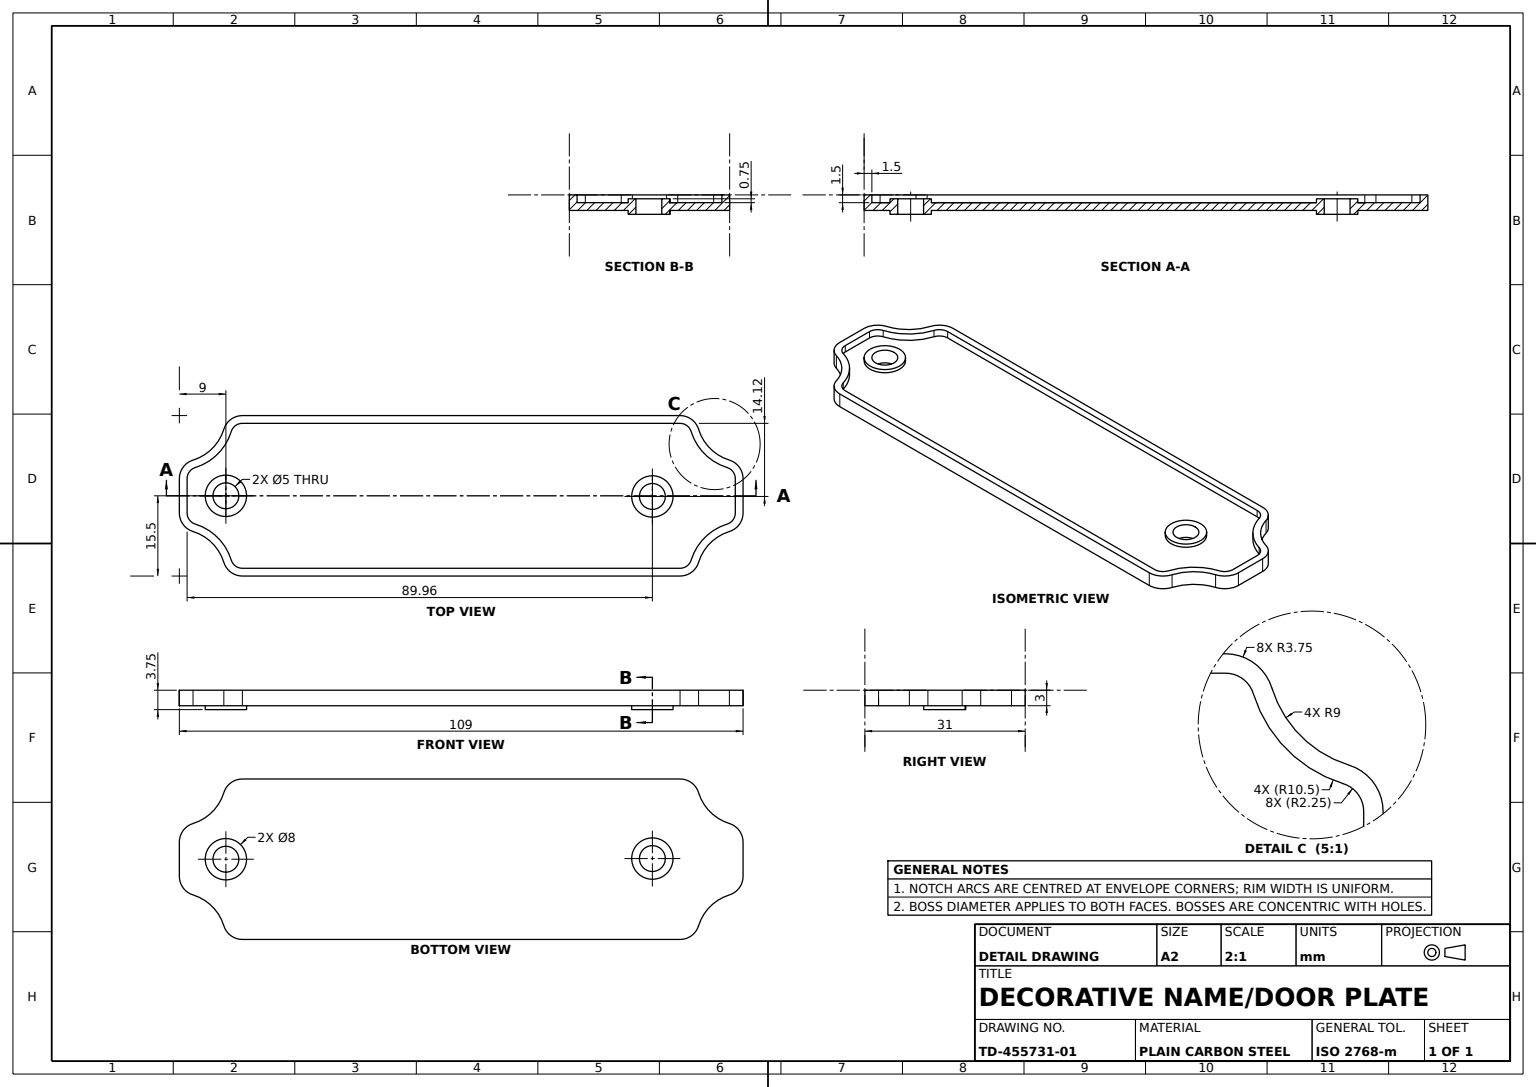
ISO-10303-21;
HEADER;
FILE_DESCRIPTION((''),'2;1');
FILE_NAME('','',(''),(''),'','','');
FILE_SCHEMA(('AUTOMOTIVE_DESIGN'));
ENDSEC;
DATA;
#1=APPLICATION_CONTEXT('');
#2=PRODUCT_CONTEXT('',#1,'mechanical');
#3=PRODUCT('','','',(#2));
#4=PRODUCT_DEFINITION_FORMATION('','',#3);
#5=PRODUCT_DEFINITION_CONTEXT('',#1,'design');
#6=PRODUCT_DEFINITION('','',#4,#5);
#7=PRODUCT_DEFINITION_SHAPE('','',#6);
#8=(LENGTH_UNIT()NAMED_UNIT(*)SI_UNIT(.MILLI.,.METRE.));
#9=(NAMED_UNIT(*)PLANE_ANGLE_UNIT()SI_UNIT($,.RADIAN.));
#10=(NAMED_UNIT(*)SI_UNIT($,.STERADIAN.)SOLID_ANGLE_UNIT());
#11=UNCERTAINTY_MEASURE_WITH_UNIT(LENGTH_MEASURE(1.E-05),#8,'distance_accuracy_value','');
#12=(GEOMETRIC_REPRESENTATION_CONTEXT(3)GLOBAL_UNCERTAINTY_ASSIGNED_CONTEXT((#11))GLOBAL_UNIT_ASSIGNED_CONTEXT((#8,#9,#10))REPRESENTATION_CONTEXT('',''));
#13=CARTESIAN_POINT('',(36.963445,-1.5,-3.876789));
#14=VERTEX_POINT('',#13);
#15=CARTESIAN_POINT('',(36.963445,-1.5,4.123211));
#16=VERTEX_POINT('',#15);
#17=CARTESIAN_POINT('',(36.963445,-1.5,0.123211));
#18=DIRECTION('',(0.,1.,0.));
#19=DIRECTION('',(0.,0.,1.));
#20=AXIS2_PLACEMENT_3D('',#17,#18,#19);
#21=CIRCLE('',#20,4.);
#22=EDGE_CURVE('',#14,#16,#21,.T.);
#23=ORIENTED_EDGE('',*,*,#22,.T.);
#24=EDGE_CURVE('',#16,#14,#21,.T.);
#25=ORIENTED_EDGE('',*,*,#24,.T.);
#26=EDGE_LOOP('',(#23,#25));
#27=FACE_BOUND('',#26,.T.);
#28=CARTESIAN_POINT('',(54.5,-1.5,-3.313942));
#29=VERTEX_POINT('',#28);
#30=CARTESIAN_POINT('',(51.852941,-1.5,-6.898077));
#31=VERTEX_POINT('',#30);
#32=CARTESIAN_POINT('',(50.75,-1.5,-3.313942));
#33=DIRECTION('',(0.,0.,-1.));
#34=AXIS2_PLACEMENT_3D('',#32,#18,#33);
#35=CIRCLE('',#34,3.75);
#36=EDGE_CURVE('',#29,#31,#35,.T.);
#37=ORIENTED_EDGE('',*,*,#36,.F.);
#38=CARTESIAN_POINT('',(54.5,-1.5,3.313942));
#39=VERTEX_POINT('',#38);
#40=VECTOR('',#33,1000.);
#41=LINE('',#28,#40);
#42=EDGE_CURVE('',#39,#29,#41,.T.);
#43=ORIENTED_EDGE('',*,*,#42,.F.);
#44=CARTESIAN_POINT('',(51.852941,-1.5,6.898077));
#45=VERTEX_POINT('',#44);
#46=CARTESIAN_POINT('',(50.75,-1.5,3.313942));
#47=AXIS2_PLACEMENT_3D('',#46,#18,#19);
#48=CIRCLE('',#47,3.75);
#49=EDGE_CURVE('',#45,#39,#48,.T.);
#50=ORIENTED_EDGE('',*,*,#49,.F.);
#51=CARTESIAN_POINT('',(45.898077,-1.5,12.852941));
#52=VERTEX_POINT('',#51);
#53=CARTESIAN_POINT('',(54.5,-1.5,15.5));
#54=DIRECTION('',(0.,-1.,0.));
#55=AXIS2_PLACEMENT_3D('',#53,#54,#19);
#56=CIRCLE('',#55,9.);
#57=EDGE_CURVE('',#52,#45,#56,.T.);
#58=ORIENTED_EDGE('',*,*,#57,.F.);
#59=CARTESIAN_POINT('',(42.313942,-1.5,15.5));
#60=VERTEX_POINT('',#59);
#61=CARTESIAN_POINT('',(42.313942,-1.5,11.75));
#62=AXIS2_PLACEMENT_3D('',#61,#18,#19);
#63=CIRCLE('',#62,3.75);
#64=EDGE_CURVE('',#60,#52,#63,.T.);
#65=ORIENTED_EDGE('',*,*,#64,.F.);
#66=CARTESIAN_POINT('',(-42.313942,-1.5,15.5));
#67=VERTEX_POINT('',#66);
#68=DIRECTION('',(1.,0.,0.));
#69=VECTOR('',#68,1000.);
#70=LINE('',#66,#69);
#71=EDGE_CURVE('',#67,#60,#70,.T.);
#72=ORIENTED_EDGE('',*,*,#71,.F.);
#73=CARTESIAN_POINT('',(-45.898077,-1.5,12.852941));
#74=VERTEX_POINT('',#73);
#75=CARTESIAN_POINT('',(-42.313942,-1.5,11.75));
#76=AXIS2_PLACEMENT_3D('',#75,#18,#19);
#77=CIRCLE('',#76,3.75);
#78=EDGE_CURVE('',#74,#67,#77,.T.);
#79=ORIENTED_EDGE('',*,*,#78,.F.);
#80=CARTESIAN_POINT('',(-51.852941,-1.5,6.898077));
#81=VERTEX_POINT('',#80);
#82=CARTESIAN_POINT('',(-54.5,-1.5,15.5));
#83=AXIS2_PLACEMENT_3D('',#82,#54,#19);
#84=CIRCLE('',#83,9.);
#85=EDGE_CURVE('',#81,#74,#84,.T.);
#86=ORIENTED_EDGE('',*,*,#85,.F.);
#87=CARTESIAN_POINT('',(-54.5,-1.5,3.313942));
#88=VERTEX_POINT('',#87);
#89=CARTESIAN_POINT('',(-50.75,-1.5,3.313942));
#90=AXIS2_PLACEMENT_3D('',#89,#18,#33);
#91=CIRCLE('',#90,3.75);
#92=EDGE_CURVE('',#88,#81,#91,.T.);
#93=ORIENTED_EDGE('',*,*,#92,.F.);
#94=CARTESIAN_POINT('',(-54.5,-1.5,-3.313942));
#95=VERTEX_POINT('',#94);
#96=VECTOR('',#19,1000.);
#97=LINE('',#94,#96);
#98=EDGE_CURVE('',#95,#88,#97,.T.);
#99=ORIENTED_EDGE('',*,*,#98,.F.);
#100=CARTESIAN_POINT('',(-51.852941,-1.5,-6.898077));
#101=VERTEX_POINT('',#100);
#102=CARTESIAN_POINT('',(-50.75,-1.5,-3.313942));
#103=AXIS2_PLACEMENT_3D('',#102,#18,#19);
#104=CIRCLE('',#103,3.75);
#105=EDGE_CURVE('',#101,#95,#104,.T.);
#106=ORIENTED_EDGE('',*,*,#105,.F.);
#107=CARTESIAN_POINT('',(-45.898077,-1.5,-12.852941));
#108=VERTEX_POINT('',#107);
#109=CARTESIAN_POINT('',(-54.5,-1.5,-15.5));
#110=AXIS2_PLACEMENT_3D('',#109,#54,#19);
#111=CIRCLE('',#110,9.);
#112=EDGE_CURVE('',#108,#101,#111,.T.);
#113=ORIENTED_EDGE('',*,*,#112,.F.);
#114=CARTESIAN_POINT('',(-42.313942,-1.5,-15.5));
#115=VERTEX_POINT('',#114);
#116=CARTESIAN_POINT('',(-42.313942,-1.5,-11.75));
#117=AXIS2_PLACEMENT_3D('',#116,#18,#19);
#118=CIRCLE('',#117,3.75);
#119=EDGE_CURVE('',#115,#108,#118,.T.);
#120=ORIENTED_EDGE('',*,*,#119,.F.);
#121=CARTESIAN_POINT('',(42.313942,-1.5,-15.5));
#122=VERTEX_POINT('',#121);
#123=DIRECTION('',(-1.,0.,0.));
#124=VECTOR('',#123,1000.);
#125=LINE('',#114,#124);
#126=EDGE_CURVE('',#122,#115,#125,.T.);
#127=ORIENTED_EDGE('',*,*,#126,.F.);
#128=CARTESIAN_POINT('',(45.898077,-1.5,-12.852941));
#129=VERTEX_POINT('',#128);
#130=CARTESIAN_POINT('',(42.313942,-1.5,-11.75));
#131=AXIS2_PLACEMENT_3D('',#130,#18,#19);
#132=CIRCLE('',#131,3.75);
#133=EDGE_CURVE('',#129,#122,#132,.T.);
#134=ORIENTED_EDGE('',*,*,#133,.F.);
#135=CARTESIAN_POINT('',(54.5,-1.5,-15.5));
#136=AXIS2_PLACEMENT_3D('',#135,#54,#19);
#137=CIRCLE('',#136,9.);
#138=EDGE_CURVE('',#31,#129,#137,.T.);
#139=ORIENTED_EDGE('',*,*,#138,.F.);
#140=EDGE_LOOP('',(#37,#43,#50,#58,#65,#72,#79,#86,#93,#99,#106,#113,#120,#127,#134,#139));
#141=FACE_OUTER_BOUND('',#140,.T.);
#142=CARTESIAN_POINT('',(-45.5,-1.5,-4.));
#143=VERTEX_POINT('',#142);
#144=CARTESIAN_POINT('',(-45.5,-1.5,4.));
#145=VERTEX_POINT('',#144);
#146=CARTESIAN_POINT('',(-45.5,-1.5,0.));
#147=AXIS2_PLACEMENT_3D('',#146,#18,#19);
#148=CIRCLE('',#147,4.);
#149=EDGE_CURVE('',#143,#145,#148,.T.);
#150=ORIENTED_EDGE('',*,*,#149,.T.);
#151=EDGE_CURVE('',#145,#143,#148,.T.);
#152=ORIENTED_EDGE('',*,*,#151,.T.);
#153=EDGE_LOOP('',(#150,#152));
#154=FACE_BOUND('',#153,.T.);
#155=PLANE('',#131);
#156=ADVANCED_FACE('',(#27,#141,#154),#155,.F.);
#157=CARTESIAN_POINT('',(-45.5,-2.25,2.5));
#158=VERTEX_POINT('',#157);
#159=CARTESIAN_POINT('',(-45.5,0.75,2.5));
#160=VERTEX_POINT('',#159);
#161=VECTOR('',#18,1000.);
#162=LINE('',#157,#161);
#163=EDGE_CURVE('',#158,#160,#162,.T.);
#164=ORIENTED_EDGE('',*,*,#163,.T.);
#165=CARTESIAN_POINT('',(-45.5,0.75,-2.5));
#166=VERTEX_POINT('',#165);
#167=CARTESIAN_POINT('',(-45.5,0.75,0.));
#168=AXIS2_PLACEMENT_3D('',#167,#18,#19);
#169=CIRCLE('',#168,2.5);
#170=EDGE_CURVE('',#160,#166,#169,.T.);
#171=ORIENTED_EDGE('',*,*,#170,.T.);
#172=CARTESIAN_POINT('',(-45.5,-2.25,-2.5));
#173=VERTEX_POINT('',#172);
#174=LINE('',#172,#161);
#175=EDGE_CURVE('',#173,#166,#174,.T.);
#176=ORIENTED_EDGE('',*,*,#175,.F.);
#177=CARTESIAN_POINT('',(-45.5,-2.25,0.));
#178=AXIS2_PLACEMENT_3D('',#177,#18,#19);
#179=CIRCLE('',#178,2.5);
#180=EDGE_CURVE('',#158,#173,#179,.T.);
#181=ORIENTED_EDGE('',*,*,#180,.F.);
#182=EDGE_LOOP('',(#164,#171,#176,#181));
#183=FACE_OUTER_BOUND('',#182,.T.);
#184=CYLINDRICAL_SURFACE('',#178,2.5);
#185=ADVANCED_FACE('',(#183),#184,.F.);
#186=CARTESIAN_POINT('',(-45.5,-2.25,-4.));
#187=VERTEX_POINT('',#186);
#188=CARTESIAN_POINT('',(-45.5,-2.25,4.));
#189=VERTEX_POINT('',#188);
#190=CIRCLE('',#178,4.);
#191=EDGE_CURVE('',#187,#189,#190,.T.);
#192=ORIENTED_EDGE('',*,*,#191,.F.);
#193=EDGE_CURVE('',#189,#187,#190,.T.);
#194=ORIENTED_EDGE('',*,*,#193,.F.);
#195=EDGE_LOOP('',(#192,#194));
#196=FACE_OUTER_BOUND('',#195,.T.);
#197=ORIENTED_EDGE('',*,*,#180,.T.);
#198=EDGE_CURVE('',#173,#158,#179,.T.);
#199=ORIENTED_EDGE('',*,*,#198,.T.);
#200=EDGE_LOOP('',(#197,#199));
#201=FACE_BOUND('',#200,.T.);
#202=PLANE('',#178);
#203=ADVANCED_FACE('',(#196,#201),#202,.F.);
#204=CARTESIAN_POINT('',(36.963445,-2.25,4.123211));
#205=VERTEX_POINT('',#204);
#206=CARTESIAN_POINT('',(36.963445,-2.25,-3.876789));
#207=VERTEX_POINT('',#206);
#208=CARTESIAN_POINT('',(36.963445,-2.25,0.123211));
#209=AXIS2_PLACEMENT_3D('',#208,#18,#19);
#210=CIRCLE('',#209,4.);
#211=EDGE_CURVE('',#205,#207,#210,.T.);
#212=ORIENTED_EDGE('',*,*,#211,.T.);
#213=LINE('',#206,#161);
#214=EDGE_CURVE('',#207,#14,#213,.T.);
#215=ORIENTED_EDGE('',*,*,#214,.T.);
#216=ORIENTED_EDGE('',*,*,#24,.F.);
#217=LINE('',#204,#161);
#218=EDGE_CURVE('',#205,#16,#217,.T.);
#219=ORIENTED_EDGE('',*,*,#218,.F.);
#220=EDGE_LOOP('',(#212,#215,#216,#219));
#221=FACE_OUTER_BOUND('',#220,.T.);
#222=CYLINDRICAL_SURFACE('',#209,4.);
#223=ADVANCED_FACE('',(#221),#222,.T.);
#224=CARTESIAN_POINT('',(-42.313942,1.5,-15.5));
#225=VERTEX_POINT('',#224);
#226=VECTOR('',#54,1000.);
#227=LINE('',#224,#226);
#228=EDGE_CURVE('',#225,#115,#227,.T.);
#229=ORIENTED_EDGE('',*,*,#228,.F.);
#230=CARTESIAN_POINT('',(42.313942,1.5,-15.5));
#231=VERTEX_POINT('',#230);
#232=LINE('',#224,#124);
#233=EDGE_CURVE('',#231,#225,#232,.T.);
#234=ORIENTED_EDGE('',*,*,#233,.F.);
#235=LINE('',#230,#226);
#236=EDGE_CURVE('',#231,#122,#235,.T.);
#237=ORIENTED_EDGE('',*,*,#236,.T.);
#238=ORIENTED_EDGE('',*,*,#126,.T.);
#239=EDGE_LOOP('',(#229,#234,#237,#238));
#240=FACE_OUTER_BOUND('',#239,.T.);
#241=AXIS2_PLACEMENT_3D('',#224,#19,#68);
#242=PLANE('',#241);
#243=ADVANCED_FACE('',(#240),#242,.F.);
#244=ORIENTED_EDGE('',*,*,#228,.T.);
#245=ORIENTED_EDGE('',*,*,#119,.T.);
#246=CARTESIAN_POINT('',(-45.898077,1.5,-12.852941));
#247=VERTEX_POINT('',#246);
#248=LINE('',#246,#226);
#249=EDGE_CURVE('',#247,#108,#248,.T.);
#250=ORIENTED_EDGE('',*,*,#249,.F.);
#251=CARTESIAN_POINT('',(-42.313942,1.5,-11.75));
#252=AXIS2_PLACEMENT_3D('',#251,#18,#19);
#253=CIRCLE('',#252,3.75);
#254=EDGE_CURVE('',#225,#247,#253,.T.);
#255=ORIENTED_EDGE('',*,*,#254,.F.);
#256=EDGE_LOOP('',(#244,#245,#250,#255));
#257=FACE_OUTER_BOUND('',#256,.T.);
#258=AXIS2_PLACEMENT_3D('',#251,#54,#33);
#259=CYLINDRICAL_SURFACE('',#258,3.75);
#260=ADVANCED_FACE('',(#257),#259,.T.);
#261=CARTESIAN_POINT('',(-53.,0.,-3.313942));
#262=VERTEX_POINT('',#261);
#263=CARTESIAN_POINT('',(-53.,1.5,-3.313942));
#264=VERTEX_POINT('',#263);
#265=LINE('',#261,#161);
#266=EDGE_CURVE('',#262,#264,#265,.T.);
#267=ORIENTED_EDGE('',*,*,#266,.T.);
#268=CARTESIAN_POINT('',(-53.,1.5,3.313942));
#269=VERTEX_POINT('',#268);
#270=LINE('',#263,#96);
#271=EDGE_CURVE('',#264,#269,#270,.T.);
#272=ORIENTED_EDGE('',*,*,#271,.T.);
#273=CARTESIAN_POINT('',(-53.,0.,3.313942));
#274=VERTEX_POINT('',#273);
#275=LINE('',#273,#161);
#276=EDGE_CURVE('',#274,#269,#275,.T.);
#277=ORIENTED_EDGE('',*,*,#276,.F.);
#278=LINE('',#261,#96);
#279=EDGE_CURVE('',#262,#274,#278,.T.);
#280=ORIENTED_EDGE('',*,*,#279,.F.);
#281=EDGE_LOOP('',(#267,#272,#277,#280));
#282=FACE_OUTER_BOUND('',#281,.T.);
#283=AXIS2_PLACEMENT_3D('',#261,#123,#19);
#284=PLANE('',#283);
#285=ADVANCED_FACE('',(#282),#284,.F.);
#286=CARTESIAN_POINT('',(36.963445,0.,-3.876789));
#287=VERTEX_POINT('',#286);
#288=CARTESIAN_POINT('',(36.963445,0.75,-3.876789));
#289=VERTEX_POINT('',#288);
#290=EDGE_CURVE('',#287,#289,#213,.T.);
#291=ORIENTED_EDGE('',*,*,#290,.T.);
#292=CARTESIAN_POINT('',(36.963445,0.75,4.123211));
#293=VERTEX_POINT('',#292);
#294=CARTESIAN_POINT('',(36.963445,0.75,0.123211));
#295=AXIS2_PLACEMENT_3D('',#294,#18,#19);
#296=CIRCLE('',#295,4.);
#297=EDGE_CURVE('',#293,#289,#296,.T.);
#298=ORIENTED_EDGE('',*,*,#297,.F.);
#299=CARTESIAN_POINT('',(36.963445,0.,4.123211));
#300=VERTEX_POINT('',#299);
#301=EDGE_CURVE('',#300,#293,#217,.T.);
#302=ORIENTED_EDGE('',*,*,#301,.F.);
#303=CARTESIAN_POINT('',(36.963445,0.,0.123211));
#304=AXIS2_PLACEMENT_3D('',#303,#18,#19);
#305=CIRCLE('',#304,4.);
#306=EDGE_CURVE('',#300,#287,#305,.T.);
#307=ORIENTED_EDGE('',*,*,#306,.T.);
#308=EDGE_LOOP('',(#291,#298,#302,#307));
#309=FACE_OUTER_BOUND('',#308,.T.);
#310=ADVANCED_FACE('',(#309),#222,.T.);
#311=EDGE_CURVE('',#289,#293,#296,.T.);
#312=ORIENTED_EDGE('',*,*,#311,.T.);
#313=ORIENTED_EDGE('',*,*,#297,.T.);
#314=EDGE_LOOP('',(#312,#313));
#315=FACE_OUTER_BOUND('',#314,.T.);
#316=CARTESIAN_POINT('',(36.963445,0.75,-2.376789));
#317=VERTEX_POINT('',#316);
#318=CARTESIAN_POINT('',(36.963445,0.75,2.623211));
#319=VERTEX_POINT('',#318);
#320=CIRCLE('',#295,2.5);
#321=EDGE_CURVE('',#317,#319,#320,.T.);
#322=ORIENTED_EDGE('',*,*,#321,.F.);
#323=EDGE_CURVE('',#319,#317,#320,.T.);
#324=ORIENTED_EDGE('',*,*,#323,.F.);
#325=EDGE_LOOP('',(#322,#324));
#326=FACE_BOUND('',#325,.T.);
#327=PLANE('',#295);
#328=ADVANCED_FACE('',(#315,#326),#327,.T.);
#329=ORIENTED_EDGE('',*,*,#311,.F.);
#330=ORIENTED_EDGE('',*,*,#290,.F.);
#331=EDGE_CURVE('',#287,#300,#305,.T.);
#332=ORIENTED_EDGE('',*,*,#331,.T.);
#333=ORIENTED_EDGE('',*,*,#301,.T.);
#334=EDGE_LOOP('',(#329,#330,#332,#333));
#335=FACE_OUTER_BOUND('',#334,.T.);
#336=ADVANCED_FACE('',(#335),#222,.T.);
#337=CARTESIAN_POINT('',(-42.313942,1.5,15.5));
#338=VERTEX_POINT('',#337);
#339=LINE('',#337,#226);
#340=EDGE_CURVE('',#338,#67,#339,.T.);
#341=ORIENTED_EDGE('',*,*,#340,.T.);
#342=ORIENTED_EDGE('',*,*,#71,.T.);
#343=CARTESIAN_POINT('',(42.313942,1.5,15.5));
#344=VERTEX_POINT('',#343);
#345=LINE('',#343,#226);
#346=EDGE_CURVE('',#344,#60,#345,.T.);
#347=ORIENTED_EDGE('',*,*,#346,.F.);
#348=LINE('',#337,#69);
#349=EDGE_CURVE('',#338,#344,#348,.T.);
#350=ORIENTED_EDGE('',*,*,#349,.F.);
#351=EDGE_LOOP('',(#341,#342,#347,#350));
#352=FACE_OUTER_BOUND('',#351,.T.);
#353=AXIS2_PLACEMENT_3D('',#337,#33,#123);
#354=PLANE('',#353);
#355=ADVANCED_FACE('',(#352),#354,.F.);
#356=CARTESIAN_POINT('',(53.,0.,-3.313942));
#357=VERTEX_POINT('',#356);
#358=CARTESIAN_POINT('',(53.,1.5,-3.313942));
#359=VERTEX_POINT('',#358);
#360=LINE('',#356,#161);
#361=EDGE_CURVE('',#357,#359,#360,.T.);
#362=ORIENTED_EDGE('',*,*,#361,.F.);
#363=CARTESIAN_POINT('',(53.,0.,3.313942));
#364=VERTEX_POINT('',#363);
#365=LINE('',#363,#40);
#366=EDGE_CURVE('',#364,#357,#365,.T.);
#367=ORIENTED_EDGE('',*,*,#366,.F.);
#368=CARTESIAN_POINT('',(53.,1.5,3.313942));
#369=VERTEX_POINT('',#368);
#370=LINE('',#363,#161);
#371=EDGE_CURVE('',#364,#369,#370,.T.);
#372=ORIENTED_EDGE('',*,*,#371,.T.);
#373=LINE('',#368,#40);
#374=EDGE_CURVE('',#369,#359,#373,.T.);
#375=ORIENTED_EDGE('',*,*,#374,.T.);
#376=EDGE_LOOP('',(#362,#367,#372,#375));
#377=FACE_OUTER_BOUND('',#376,.T.);
#378=AXIS2_PLACEMENT_3D('',#363,#68,#33);
#379=PLANE('',#378);
#380=ADVANCED_FACE('',(#377),#379,.F.);
#381=CARTESIAN_POINT('',(-51.852941,1.5,-6.898077));
#382=VERTEX_POINT('',#381);
#383=CARTESIAN_POINT('',(-54.5,1.5,-3.313942));
#384=VERTEX_POINT('',#383);
#385=CARTESIAN_POINT('',(-50.75,1.5,-3.313942));
#386=AXIS2_PLACEMENT_3D('',#385,#18,#19);
#387=CIRCLE('',#386,3.75);
#388=EDGE_CURVE('',#382,#384,#387,.T.);
#389=ORIENTED_EDGE('',*,*,#388,.T.);
#390=CARTESIAN_POINT('',(-54.5,1.5,3.313942));
#391=VERTEX_POINT('',#390);
#392=LINE('',#383,#96);
#393=EDGE_CURVE('',#384,#391,#392,.T.);
#394=ORIENTED_EDGE('',*,*,#393,.T.);
#395=CARTESIAN_POINT('',(-51.852941,1.5,6.898077));
#396=VERTEX_POINT('',#395);
#397=CARTESIAN_POINT('',(-50.75,1.5,3.313942));
#398=AXIS2_PLACEMENT_3D('',#397,#18,#33);
#399=CIRCLE('',#398,3.75);
#400=EDGE_CURVE('',#391,#396,#399,.T.);
#401=ORIENTED_EDGE('',*,*,#400,.T.);
#402=CARTESIAN_POINT('',(-45.898077,1.5,12.852941));
#403=VERTEX_POINT('',#402);
#404=CARTESIAN_POINT('',(-54.5,1.5,15.5));
#405=AXIS2_PLACEMENT_3D('',#404,#54,#19);
#406=CIRCLE('',#405,9.);
#407=EDGE_CURVE('',#396,#403,#406,.T.);
#408=ORIENTED_EDGE('',*,*,#407,.T.);
#409=CARTESIAN_POINT('',(-42.313942,1.5,11.75));
#410=AXIS2_PLACEMENT_3D('',#409,#18,#19);
#411=CIRCLE('',#410,3.75);
#412=EDGE_CURVE('',#403,#338,#411,.T.);
#413=ORIENTED_EDGE('',*,*,#412,.T.);
#414=ORIENTED_EDGE('',*,*,#349,.T.);
#415=CARTESIAN_POINT('',(45.898077,1.5,12.852941));
#416=VERTEX_POINT('',#415);
#417=CARTESIAN_POINT('',(42.313942,1.5,11.75));
#418=AXIS2_PLACEMENT_3D('',#417,#18,#19);
#419=CIRCLE('',#418,3.75);
#420=EDGE_CURVE('',#344,#416,#419,.T.);
#421=ORIENTED_EDGE('',*,*,#420,.T.);
#422=CARTESIAN_POINT('',(51.852941,1.5,6.898077));
#423=VERTEX_POINT('',#422);
#424=CARTESIAN_POINT('',(54.5,1.5,15.5));
#425=AXIS2_PLACEMENT_3D('',#424,#54,#19);
#426=CIRCLE('',#425,9.);
#427=EDGE_CURVE('',#416,#423,#426,.T.);
#428=ORIENTED_EDGE('',*,*,#427,.T.);
#429=CARTESIAN_POINT('',(54.5,1.5,3.313942));
#430=VERTEX_POINT('',#429);
#431=CARTESIAN_POINT('',(50.75,1.5,3.313942));
#432=AXIS2_PLACEMENT_3D('',#431,#18,#19);
#433=CIRCLE('',#432,3.75);
#434=EDGE_CURVE('',#423,#430,#433,.T.);
#435=ORIENTED_EDGE('',*,*,#434,.T.);
#436=CARTESIAN_POINT('',(54.5,1.5,-3.313942));
#437=VERTEX_POINT('',#436);
#438=LINE('',#436,#40);
#439=EDGE_CURVE('',#430,#437,#438,.T.);
#440=ORIENTED_EDGE('',*,*,#439,.T.);
#441=CARTESIAN_POINT('',(51.852941,1.5,-6.898077));
#442=VERTEX_POINT('',#441);
#443=CARTESIAN_POINT('',(50.75,1.5,-3.313942));
#444=AXIS2_PLACEMENT_3D('',#443,#18,#33);
#445=CIRCLE('',#444,3.75);
#446=EDGE_CURVE('',#437,#442,#445,.T.);
#447=ORIENTED_EDGE('',*,*,#446,.T.);
#448=CARTESIAN_POINT('',(45.898077,1.5,-12.852941));
#449=VERTEX_POINT('',#448);
#450=CARTESIAN_POINT('',(54.5,1.5,-15.5));
#451=AXIS2_PLACEMENT_3D('',#450,#54,#19);
#452=CIRCLE('',#451,9.);
#453=EDGE_CURVE('',#442,#449,#452,.T.);
#454=ORIENTED_EDGE('',*,*,#453,.T.);
#455=CARTESIAN_POINT('',(42.313942,1.5,-11.75));
#456=AXIS2_PLACEMENT_3D('',#455,#18,#19);
#457=CIRCLE('',#456,3.75);
#458=EDGE_CURVE('',#449,#231,#457,.T.);
#459=ORIENTED_EDGE('',*,*,#458,.T.);
#460=ORIENTED_EDGE('',*,*,#233,.T.);
#461=ORIENTED_EDGE('',*,*,#254,.T.);
#462=CARTESIAN_POINT('',(-54.5,1.5,-15.5));
#463=AXIS2_PLACEMENT_3D('',#462,#54,#19);
#464=CIRCLE('',#463,9.);
#465=EDGE_CURVE('',#247,#382,#464,.T.);
#466=ORIENTED_EDGE('',*,*,#465,.T.);
#467=EDGE_LOOP('',(#389,#394,#401,#408,#413,#414,#421,#428,#435,#440,#447,#454,#459,#460,#461,#466));
#468=FACE_OUTER_BOUND('',#467,.T.);
#469=CARTESIAN_POINT('',(-51.411765,1.5,5.464423));
#470=VERTEX_POINT('',#469);
#471=AXIS2_PLACEMENT_3D('',#397,#18,#19);
#472=CIRCLE('',#471,2.25);
#473=EDGE_CURVE('',#269,#470,#472,.T.);
#474=ORIENTED_EDGE('',*,*,#473,.F.);
#475=ORIENTED_EDGE('',*,*,#271,.F.);
#476=CARTESIAN_POINT('',(-51.411765,1.5,-5.464423));
#477=VERTEX_POINT('',#476);
#478=CIRCLE('',#386,2.25);
#479=EDGE_CURVE('',#477,#264,#478,.T.);
#480=ORIENTED_EDGE('',*,*,#479,.F.);
#481=CARTESIAN_POINT('',(-44.464423,1.5,-12.411765));
#482=VERTEX_POINT('',#481);
#483=CIRCLE('',#463,10.5);
#484=EDGE_CURVE('',#482,#477,#483,.T.);
#485=ORIENTED_EDGE('',*,*,#484,.F.);
#486=CARTESIAN_POINT('',(-42.313942,1.5,-14.));
#487=VERTEX_POINT('',#486);
#488=CIRCLE('',#252,2.25);
#489=EDGE_CURVE('',#487,#482,#488,.T.);
#490=ORIENTED_EDGE('',*,*,#489,.F.);
#491=CARTESIAN_POINT('',(42.313942,1.5,-14.));
#492=VERTEX_POINT('',#491);
#493=LINE('',#491,#124);
#494=EDGE_CURVE('',#492,#487,#493,.T.);
#495=ORIENTED_EDGE('',*,*,#494,.F.);
#496=CARTESIAN_POINT('',(44.464423,1.5,-12.411765));
#497=VERTEX_POINT('',#496);
#498=CIRCLE('',#456,2.25);
#499=EDGE_CURVE('',#497,#492,#498,.T.);
#500=ORIENTED_EDGE('',*,*,#499,.F.);
#501=CARTESIAN_POINT('',(51.411765,1.5,-5.464423));
#502=VERTEX_POINT('',#501);
#503=CIRCLE('',#451,10.5);
#504=EDGE_CURVE('',#502,#497,#503,.T.);
#505=ORIENTED_EDGE('',*,*,#504,.F.);
#506=AXIS2_PLACEMENT_3D('',#443,#18,#19);
#507=CIRCLE('',#506,2.25);
#508=EDGE_CURVE('',#359,#502,#507,.T.);
#509=ORIENTED_EDGE('',*,*,#508,.F.);
#510=ORIENTED_EDGE('',*,*,#374,.F.);
#511=CARTESIAN_POINT('',(51.411765,1.5,5.464423));
#512=VERTEX_POINT('',#511);
#513=CIRCLE('',#432,2.25);
#514=EDGE_CURVE('',#512,#369,#513,.T.);
#515=ORIENTED_EDGE('',*,*,#514,.F.);
#516=CARTESIAN_POINT('',(44.464423,1.5,12.411765));
#517=VERTEX_POINT('',#516);
#518=CIRCLE('',#425,10.5);
#519=EDGE_CURVE('',#517,#512,#518,.T.);
#520=ORIENTED_EDGE('',*,*,#519,.F.);
#521=CARTESIAN_POINT('',(42.313942,1.5,14.));
#522=VERTEX_POINT('',#521);
#523=CIRCLE('',#418,2.25);
#524=EDGE_CURVE('',#522,#517,#523,.T.);
#525=ORIENTED_EDGE('',*,*,#524,.F.);
#526=CARTESIAN_POINT('',(-42.313942,1.5,14.));
#527=VERTEX_POINT('',#526);
#528=LINE('',#526,#69);
#529=EDGE_CURVE('',#527,#522,#528,.T.);
#530=ORIENTED_EDGE('',*,*,#529,.F.);
#531=CARTESIAN_POINT('',(-44.464423,1.5,12.411765));
#532=VERTEX_POINT('',#531);
#533=CIRCLE('',#410,2.25);
#534=EDGE_CURVE('',#532,#527,#533,.T.);
#535=ORIENTED_EDGE('',*,*,#534,.F.);
#536=CIRCLE('',#405,10.5);
#537=EDGE_CURVE('',#470,#532,#536,.T.);
#538=ORIENTED_EDGE('',*,*,#537,.F.);
#539=EDGE_LOOP('',(#474,#475,#480,#485,#490,#495,#500,#505,#509,#510,#515,#520,#525,#530,#535,#538));
#540=FACE_BOUND('',#539,.T.);
#541=PLANE('',#456);
#542=ADVANCED_FACE('',(#468,#540),#541,.T.);
#543=ORIENTED_EDGE('',*,*,#439,.F.);
#544=LINE('',#429,#226);
#545=EDGE_CURVE('',#430,#39,#544,.T.);
#546=ORIENTED_EDGE('',*,*,#545,.T.);
#547=ORIENTED_EDGE('',*,*,#42,.T.);
#548=LINE('',#436,#226);
#549=EDGE_CURVE('',#437,#29,#548,.T.);
#550=ORIENTED_EDGE('',*,*,#549,.F.);
#551=EDGE_LOOP('',(#543,#546,#547,#550));
#552=FACE_OUTER_BOUND('',#551,.T.);
#553=AXIS2_PLACEMENT_3D('',#436,#123,#19);
#554=PLANE('',#553);
#555=ADVANCED_FACE('',(#552),#554,.F.);
#556=CARTESIAN_POINT('',(-44.464423,0.,-12.411765));
#557=VERTEX_POINT('',#556);
#558=LINE('',#556,#161);
#559=EDGE_CURVE('',#557,#482,#558,.T.);
#560=ORIENTED_EDGE('',*,*,#559,.T.);
#561=ORIENTED_EDGE('',*,*,#484,.T.);
#562=CARTESIAN_POINT('',(-51.411765,0.,-5.464423));
#563=VERTEX_POINT('',#562);
#564=LINE('',#562,#161);
#565=EDGE_CURVE('',#563,#477,#564,.T.);
#566=ORIENTED_EDGE('',*,*,#565,.F.);
#567=CARTESIAN_POINT('',(-54.5,0.,-15.5));
#568=AXIS2_PLACEMENT_3D('',#567,#54,#19);
#569=CIRCLE('',#568,10.5);
#570=EDGE_CURVE('',#557,#563,#569,.T.);
#571=ORIENTED_EDGE('',*,*,#570,.F.);
#572=EDGE_LOOP('',(#560,#561,#566,#571));
#573=FACE_OUTER_BOUND('',#572,.T.);
#574=AXIS2_PLACEMENT_3D('',#567,#18,#19);
#575=CYLINDRICAL_SURFACE('',#574,10.5);
#576=ADVANCED_FACE('',(#573),#575,.T.);
#577=ORIENTED_EDGE('',*,*,#524,.T.);
#578=CARTESIAN_POINT('',(44.464423,0.,12.411765));
#579=VERTEX_POINT('',#578);
#580=LINE('',#578,#161);
#581=EDGE_CURVE('',#579,#517,#580,.T.);
#582=ORIENTED_EDGE('',*,*,#581,.F.);
#583=CARTESIAN_POINT('',(42.313942,0.,14.));
#584=VERTEX_POINT('',#583);
#585=CARTESIAN_POINT('',(42.313942,0.,11.75));
#586=AXIS2_PLACEMENT_3D('',#585,#18,#19);
#587=CIRCLE('',#586,2.25);
#588=EDGE_CURVE('',#584,#579,#587,.T.);
#589=ORIENTED_EDGE('',*,*,#588,.F.);
#590=LINE('',#583,#161);
#591=EDGE_CURVE('',#584,#522,#590,.T.);
#592=ORIENTED_EDGE('',*,*,#591,.T.);
#593=EDGE_LOOP('',(#577,#582,#589,#592));
#594=FACE_OUTER_BOUND('',#593,.T.);
#595=CYLINDRICAL_SURFACE('',#586,2.25);
#596=ADVANCED_FACE('',(#594),#595,.F.);
#597=CARTESIAN_POINT('',(-45.5,0.,4.));
#598=VERTEX_POINT('',#597);
#599=CARTESIAN_POINT('',(-45.5,0.75,4.));
#600=VERTEX_POINT('',#599);
#601=LINE('',#188,#161);
#602=EDGE_CURVE('',#598,#600,#601,.T.);
#603=ORIENTED_EDGE('',*,*,#602,.F.);
#604=CARTESIAN_POINT('',(-45.5,0.,-4.));
#605=VERTEX_POINT('',#604);
#606=CARTESIAN_POINT('',(-45.5,0.,0.));
#607=AXIS2_PLACEMENT_3D('',#606,#18,#19);
#608=CIRCLE('',#607,4.);
#609=EDGE_CURVE('',#598,#605,#608,.T.);
#610=ORIENTED_EDGE('',*,*,#609,.T.);
#611=CARTESIAN_POINT('',(-45.5,0.75,-4.));
#612=VERTEX_POINT('',#611);
#613=LINE('',#186,#161);
#614=EDGE_CURVE('',#605,#612,#613,.T.);
#615=ORIENTED_EDGE('',*,*,#614,.T.);
#616=CIRCLE('',#168,4.);
#617=EDGE_CURVE('',#600,#612,#616,.T.);
#618=ORIENTED_EDGE('',*,*,#617,.F.);
#619=EDGE_LOOP('',(#603,#610,#615,#618));
#620=FACE_OUTER_BOUND('',#619,.T.);
#621=CYLINDRICAL_SURFACE('',#178,4.);
#622=ADVANCED_FACE('',(#620),#621,.T.);
#623=ORIENTED_EDGE('',*,*,#85,.T.);
#624=LINE('',#402,#226);
#625=EDGE_CURVE('',#403,#74,#624,.T.);
#626=ORIENTED_EDGE('',*,*,#625,.F.);
#627=ORIENTED_EDGE('',*,*,#407,.F.);
#628=LINE('',#395,#226);
#629=EDGE_CURVE('',#396,#81,#628,.T.);
#630=ORIENTED_EDGE('',*,*,#629,.T.);
#631=EDGE_LOOP('',(#623,#626,#627,#630));
#632=FACE_OUTER_BOUND('',#631,.T.);
#633=AXIS2_PLACEMENT_3D('',#404,#54,#33);
#634=CYLINDRICAL_SURFACE('',#633,9.);
#635=ADVANCED_FACE('',(#632),#634,.F.);
#636=LINE('',#448,#226);
#637=EDGE_CURVE('',#449,#129,#636,.T.);
#638=ORIENTED_EDGE('',*,*,#637,.T.);
#639=ORIENTED_EDGE('',*,*,#133,.T.);
#640=ORIENTED_EDGE('',*,*,#236,.F.);
#641=ORIENTED_EDGE('',*,*,#458,.F.);
#642=EDGE_LOOP('',(#638,#639,#640,#641));
#643=FACE_OUTER_BOUND('',#642,.T.);
#644=AXIS2_PLACEMENT_3D('',#455,#54,#33);
#645=CYLINDRICAL_SURFACE('',#644,3.75);
#646=ADVANCED_FACE('',(#643),#645,.T.);
#647=ORIENTED_EDGE('',*,*,#446,.F.);
#648=ORIENTED_EDGE('',*,*,#549,.T.);
#649=ORIENTED_EDGE('',*,*,#36,.T.);
#650=LINE('',#441,#226);
#651=EDGE_CURVE('',#442,#31,#650,.T.);
#652=ORIENTED_EDGE('',*,*,#651,.F.);
#653=EDGE_LOOP('',(#647,#648,#649,#652));
#654=FACE_OUTER_BOUND('',#653,.T.);
#655=AXIS2_PLACEMENT_3D('',#443,#54,#33);
#656=CYLINDRICAL_SURFACE('',#655,3.75);
#657=ADVANCED_FACE('',(#654),#656,.T.);
#658=EDGE_CURVE('',#187,#143,#613,.T.);
#659=ORIENTED_EDGE('',*,*,#658,.F.);
#660=ORIENTED_EDGE('',*,*,#191,.T.);
#661=EDGE_CURVE('',#189,#145,#601,.T.);
#662=ORIENTED_EDGE('',*,*,#661,.T.);
#663=ORIENTED_EDGE('',*,*,#149,.F.);
#664=EDGE_LOOP('',(#659,#660,#662,#663));
#665=FACE_OUTER_BOUND('',#664,.T.);
#666=ADVANCED_FACE('',(#665),#621,.T.);
#667=CARTESIAN_POINT('',(51.411765,0.,5.464423));
#668=VERTEX_POINT('',#667);
#669=CARTESIAN_POINT('',(54.5,0.,15.5));
#670=AXIS2_PLACEMENT_3D('',#669,#54,#19);
#671=CIRCLE('',#670,10.5);
#672=EDGE_CURVE('',#579,#668,#671,.T.);
#673=ORIENTED_EDGE('',*,*,#672,.F.);
#674=ORIENTED_EDGE('',*,*,#581,.T.);
#675=ORIENTED_EDGE('',*,*,#519,.T.);
#676=LINE('',#667,#161);
#677=EDGE_CURVE('',#668,#512,#676,.T.);
#678=ORIENTED_EDGE('',*,*,#677,.F.);
#679=EDGE_LOOP('',(#673,#674,#675,#678));
#680=FACE_OUTER_BOUND('',#679,.T.);
#681=AXIS2_PLACEMENT_3D('',#669,#18,#19);
#682=CYLINDRICAL_SURFACE('',#681,10.5);
#683=ADVANCED_FACE('',(#680),#682,.T.);
#684=CARTESIAN_POINT('',(51.411765,0.,-5.464423));
#685=VERTEX_POINT('',#684);
#686=CARTESIAN_POINT('',(50.75,0.,-3.313942));
#687=AXIS2_PLACEMENT_3D('',#686,#18,#19);
#688=CIRCLE('',#687,2.25);
#689=EDGE_CURVE('',#357,#685,#688,.T.);
#690=ORIENTED_EDGE('',*,*,#689,.F.);
#691=ORIENTED_EDGE('',*,*,#361,.T.);
#692=ORIENTED_EDGE('',*,*,#508,.T.);
#693=LINE('',#684,#161);
#694=EDGE_CURVE('',#685,#502,#693,.T.);
#695=ORIENTED_EDGE('',*,*,#694,.F.);
#696=EDGE_LOOP('',(#690,#691,#692,#695));
#697=FACE_OUTER_BOUND('',#696,.T.);
#698=CYLINDRICAL_SURFACE('',#687,2.25);
#699=ADVANCED_FACE('',(#697),#698,.F.);
#700=ORIENTED_EDGE('',*,*,#346,.T.);
#701=ORIENTED_EDGE('',*,*,#64,.T.);
#702=LINE('',#415,#226);
#703=EDGE_CURVE('',#416,#52,#702,.T.);
#704=ORIENTED_EDGE('',*,*,#703,.F.);
#705=ORIENTED_EDGE('',*,*,#420,.F.);
#706=EDGE_LOOP('',(#700,#701,#704,#705));
#707=FACE_OUTER_BOUND('',#706,.T.);
#708=AXIS2_PLACEMENT_3D('',#417,#54,#33);
#709=CYLINDRICAL_SURFACE('',#708,3.75);
#710=ADVANCED_FACE('',(#707),#709,.T.);
#711=CARTESIAN_POINT('',(36.963445,-2.25,-2.376789));
#712=VERTEX_POINT('',#711);
#713=LINE('',#711,#161);
#714=EDGE_CURVE('',#712,#317,#713,.T.);
#715=ORIENTED_EDGE('',*,*,#714,.T.);
#716=ORIENTED_EDGE('',*,*,#321,.T.);
#717=CARTESIAN_POINT('',(36.963445,-2.25,2.623211));
#718=VERTEX_POINT('',#717);
#719=LINE('',#717,#161);
#720=EDGE_CURVE('',#718,#319,#719,.T.);
#721=ORIENTED_EDGE('',*,*,#720,.F.);
#722=CIRCLE('',#209,2.5);
#723=EDGE_CURVE('',#712,#718,#722,.T.);
#724=ORIENTED_EDGE('',*,*,#723,.F.);
#725=EDGE_LOOP('',(#715,#716,#721,#724));
#726=FACE_OUTER_BOUND('',#725,.T.);
#727=CYLINDRICAL_SURFACE('',#209,2.5);
#728=ADVANCED_FACE('',(#726),#727,.F.);
#729=CARTESIAN_POINT('',(44.464423,0.,-12.411765));
#730=VERTEX_POINT('',#729);
#731=LINE('',#729,#161);
#732=EDGE_CURVE('',#730,#497,#731,.T.);
#733=ORIENTED_EDGE('',*,*,#732,.F.);
#734=CARTESIAN_POINT('',(54.5,0.,-15.5));
#735=AXIS2_PLACEMENT_3D('',#734,#54,#19);
#736=CIRCLE('',#735,10.5);
#737=EDGE_CURVE('',#685,#730,#736,.T.);
#738=ORIENTED_EDGE('',*,*,#737,.F.);
#739=ORIENTED_EDGE('',*,*,#694,.T.);
#740=ORIENTED_EDGE('',*,*,#504,.T.);
#741=EDGE_LOOP('',(#733,#738,#739,#740));
#742=FACE_OUTER_BOUND('',#741,.T.);
#743=AXIS2_PLACEMENT_3D('',#734,#18,#19);
#744=CYLINDRICAL_SURFACE('',#743,10.5);
#745=ADVANCED_FACE('',(#742),#744,.T.);
#746=ORIENTED_EDGE('',*,*,#138,.T.);
#747=ORIENTED_EDGE('',*,*,#637,.F.);
#748=ORIENTED_EDGE('',*,*,#453,.F.);
#749=ORIENTED_EDGE('',*,*,#651,.T.);
#750=EDGE_LOOP('',(#746,#747,#748,#749));
#751=FACE_OUTER_BOUND('',#750,.T.);
#752=AXIS2_PLACEMENT_3D('',#450,#54,#33);
#753=CYLINDRICAL_SURFACE('',#752,9.);
#754=ADVANCED_FACE('',(#751),#753,.F.);
#755=EDGE_CURVE('',#605,#598,#608,.T.);
#756=ORIENTED_EDGE('',*,*,#755,.T.);
#757=ORIENTED_EDGE('',*,*,#602,.T.);
#758=EDGE_CURVE('',#612,#600,#616,.T.);
#759=ORIENTED_EDGE('',*,*,#758,.F.);
#760=ORIENTED_EDGE('',*,*,#614,.F.);
#761=EDGE_LOOP('',(#756,#757,#759,#760));
#762=FACE_OUTER_BOUND('',#761,.T.);
#763=ADVANCED_FACE('',(#762),#621,.T.);
#764=CARTESIAN_POINT('',(-42.313942,0.,-14.));
#765=VERTEX_POINT('',#764);
#766=CARTESIAN_POINT('',(-42.313942,0.,-11.75));
#767=AXIS2_PLACEMENT_3D('',#766,#18,#19);
#768=CIRCLE('',#767,2.25);
#769=EDGE_CURVE('',#765,#557,#768,.T.);
#770=ORIENTED_EDGE('',*,*,#769,.F.);
#771=LINE('',#764,#161);
#772=EDGE_CURVE('',#765,#487,#771,.T.);
#773=ORIENTED_EDGE('',*,*,#772,.T.);
#774=ORIENTED_EDGE('',*,*,#489,.T.);
#775=ORIENTED_EDGE('',*,*,#559,.F.);
#776=EDGE_LOOP('',(#770,#773,#774,#775));
#777=FACE_OUTER_BOUND('',#776,.T.);
#778=CYLINDRICAL_SURFACE('',#767,2.25);
#779=ADVANCED_FACE('',(#777),#778,.F.);
#780=ORIENTED_EDGE('',*,*,#427,.F.);
#781=ORIENTED_EDGE('',*,*,#703,.T.);
#782=ORIENTED_EDGE('',*,*,#57,.T.);
#783=LINE('',#422,#226);
#784=EDGE_CURVE('',#423,#45,#783,.T.);
#785=ORIENTED_EDGE('',*,*,#784,.F.);
#786=EDGE_LOOP('',(#780,#781,#782,#785));
#787=FACE_OUTER_BOUND('',#786,.T.);
#788=AXIS2_PLACEMENT_3D('',#424,#54,#33);
#789=CYLINDRICAL_SURFACE('',#788,9.);
#790=ADVANCED_FACE('',(#787),#789,.F.);
#791=LINE('',#381,#226);
#792=EDGE_CURVE('',#382,#101,#791,.T.);
#793=ORIENTED_EDGE('',*,*,#792,.T.);
#794=ORIENTED_EDGE('',*,*,#105,.T.);
#795=LINE('',#383,#226);
#796=EDGE_CURVE('',#384,#95,#795,.T.);
#797=ORIENTED_EDGE('',*,*,#796,.F.);
#798=ORIENTED_EDGE('',*,*,#388,.F.);
#799=EDGE_LOOP('',(#793,#794,#797,#798));
#800=FACE_OUTER_BOUND('',#799,.T.);
#801=AXIS2_PLACEMENT_3D('',#385,#54,#33);
#802=CYLINDRICAL_SURFACE('',#801,3.75);
#803=ADVANCED_FACE('',(#800),#802,.T.);
#804=ORIENTED_EDGE('',*,*,#49,.T.);
#805=ORIENTED_EDGE('',*,*,#545,.F.);
#806=ORIENTED_EDGE('',*,*,#434,.F.);
#807=ORIENTED_EDGE('',*,*,#784,.T.);
#808=EDGE_LOOP('',(#804,#805,#806,#807));
#809=FACE_OUTER_BOUND('',#808,.T.);
#810=AXIS2_PLACEMENT_3D('',#431,#54,#33);
#811=CYLINDRICAL_SURFACE('',#810,3.75);
#812=ADVANCED_FACE('',(#809),#811,.T.);
#813=ORIENTED_EDGE('',*,*,#723,.T.);
#814=EDGE_CURVE('',#718,#712,#722,.T.);
#815=ORIENTED_EDGE('',*,*,#814,.T.);
#816=EDGE_LOOP('',(#813,#815));
#817=FACE_BOUND('',#816,.T.);
#818=EDGE_CURVE('',#207,#205,#210,.T.);
#819=ORIENTED_EDGE('',*,*,#818,.F.);
#820=ORIENTED_EDGE('',*,*,#211,.F.);
#821=EDGE_LOOP('',(#819,#820));
#822=FACE_OUTER_BOUND('',#821,.T.);
#823=PLANE('',#209);
#824=ADVANCED_FACE('',(#817,#822),#823,.F.);
#825=ORIENTED_EDGE('',*,*,#814,.F.);
#826=ORIENTED_EDGE('',*,*,#720,.T.);
#827=ORIENTED_EDGE('',*,*,#323,.T.);
#828=ORIENTED_EDGE('',*,*,#714,.F.);
#829=EDGE_LOOP('',(#825,#826,#827,#828));
#830=FACE_OUTER_BOUND('',#829,.T.);
#831=ADVANCED_FACE('',(#830),#727,.F.);
#832=ORIENTED_EDGE('',*,*,#218,.T.);
#833=ORIENTED_EDGE('',*,*,#22,.F.);
#834=ORIENTED_EDGE('',*,*,#214,.F.);
#835=ORIENTED_EDGE('',*,*,#818,.T.);
#836=EDGE_LOOP('',(#832,#833,#834,#835));
#837=FACE_OUTER_BOUND('',#836,.T.);
#838=ADVANCED_FACE('',(#837),#222,.T.);
#839=ORIENTED_EDGE('',*,*,#393,.F.);
#840=ORIENTED_EDGE('',*,*,#796,.T.);
#841=ORIENTED_EDGE('',*,*,#98,.T.);
#842=LINE('',#390,#226);
#843=EDGE_CURVE('',#391,#88,#842,.T.);
#844=ORIENTED_EDGE('',*,*,#843,.F.);
#845=EDGE_LOOP('',(#839,#840,#841,#844));
#846=FACE_OUTER_BOUND('',#845,.T.);
#847=AXIS2_PLACEMENT_3D('',#383,#68,#33);
#848=PLANE('',#847);
#849=ADVANCED_FACE('',(#846),#848,.F.);
#850=CARTESIAN_POINT('',(-51.411765,0.,5.464423));
#851=VERTEX_POINT('',#850);
#852=LINE('',#850,#161);
#853=EDGE_CURVE('',#851,#470,#852,.T.);
#854=ORIENTED_EDGE('',*,*,#853,.T.);
#855=ORIENTED_EDGE('',*,*,#537,.T.);
#856=CARTESIAN_POINT('',(-44.464423,0.,12.411765));
#857=VERTEX_POINT('',#856);
#858=LINE('',#856,#161);
#859=EDGE_CURVE('',#857,#532,#858,.T.);
#860=ORIENTED_EDGE('',*,*,#859,.F.);
#861=CARTESIAN_POINT('',(-54.5,0.,15.5));
#862=AXIS2_PLACEMENT_3D('',#861,#54,#19);
#863=CIRCLE('',#862,10.5);
#864=EDGE_CURVE('',#851,#857,#863,.T.);
#865=ORIENTED_EDGE('',*,*,#864,.F.);
#866=EDGE_LOOP('',(#854,#855,#860,#865));
#867=FACE_OUTER_BOUND('',#866,.T.);
#868=AXIS2_PLACEMENT_3D('',#861,#18,#19);
#869=CYLINDRICAL_SURFACE('',#868,10.5);
#870=ADVANCED_FACE('',(#867),#869,.T.);
#871=ORIENTED_EDGE('',*,*,#198,.F.);
#872=ORIENTED_EDGE('',*,*,#175,.T.);
#873=EDGE_CURVE('',#166,#160,#169,.T.);
#874=ORIENTED_EDGE('',*,*,#873,.T.);
#875=ORIENTED_EDGE('',*,*,#163,.F.);
#876=EDGE_LOOP('',(#871,#872,#874,#875));
#877=FACE_OUTER_BOUND('',#876,.T.);
#878=ADVANCED_FACE('',(#877),#184,.F.);
#879=ORIENTED_EDGE('',*,*,#514,.T.);
#880=ORIENTED_EDGE('',*,*,#371,.F.);
#881=CARTESIAN_POINT('',(50.75,0.,3.313942));
#882=AXIS2_PLACEMENT_3D('',#881,#18,#19);
#883=CIRCLE('',#882,2.25);
#884=EDGE_CURVE('',#668,#364,#883,.T.);
#885=ORIENTED_EDGE('',*,*,#884,.F.);
#886=ORIENTED_EDGE('',*,*,#677,.T.);
#887=EDGE_LOOP('',(#879,#880,#885,#886));
#888=FACE_OUTER_BOUND('',#887,.T.);
#889=CYLINDRICAL_SURFACE('',#882,2.25);
#890=ADVANCED_FACE('',(#888),#889,.F.);
#891=ORIENTED_EDGE('',*,*,#400,.F.);
#892=ORIENTED_EDGE('',*,*,#843,.T.);
#893=ORIENTED_EDGE('',*,*,#92,.T.);
#894=ORIENTED_EDGE('',*,*,#629,.F.);
#895=EDGE_LOOP('',(#891,#892,#893,#894));
#896=FACE_OUTER_BOUND('',#895,.T.);
#897=AXIS2_PLACEMENT_3D('',#397,#54,#33);
#898=CYLINDRICAL_SURFACE('',#897,3.75);
#899=ADVANCED_FACE('',(#896),#898,.T.);
#900=ORIENTED_EDGE('',*,*,#617,.T.);
#901=ORIENTED_EDGE('',*,*,#758,.T.);
#902=EDGE_LOOP('',(#900,#901));
#903=FACE_OUTER_BOUND('',#902,.T.);
#904=ORIENTED_EDGE('',*,*,#170,.F.);
#905=ORIENTED_EDGE('',*,*,#873,.F.);
#906=EDGE_LOOP('',(#904,#905));
#907=FACE_BOUND('',#906,.T.);
#908=PLANE('',#168);
#909=ADVANCED_FACE('',(#903,#907),#908,.T.);
#910=ORIENTED_EDGE('',*,*,#658,.T.);
#911=ORIENTED_EDGE('',*,*,#151,.F.);
#912=ORIENTED_EDGE('',*,*,#661,.F.);
#913=ORIENTED_EDGE('',*,*,#193,.T.);
#914=EDGE_LOOP('',(#910,#911,#912,#913));
#915=FACE_OUTER_BOUND('',#914,.T.);
#916=ADVANCED_FACE('',(#915),#621,.T.);
#917=ORIENTED_EDGE('',*,*,#465,.F.);
#918=ORIENTED_EDGE('',*,*,#249,.T.);
#919=ORIENTED_EDGE('',*,*,#112,.T.);
#920=ORIENTED_EDGE('',*,*,#792,.F.);
#921=EDGE_LOOP('',(#917,#918,#919,#920));
#922=FACE_OUTER_BOUND('',#921,.T.);
#923=AXIS2_PLACEMENT_3D('',#462,#54,#33);
#924=CYLINDRICAL_SURFACE('',#923,9.);
#925=ADVANCED_FACE('',(#922),#924,.F.);
#926=ORIENTED_EDGE('',*,*,#279,.T.);
#927=CARTESIAN_POINT('',(-50.75,0.,3.313942));
#928=AXIS2_PLACEMENT_3D('',#927,#18,#19);
#929=CIRCLE('',#928,2.25);
#930=EDGE_CURVE('',#274,#851,#929,.T.);
#931=ORIENTED_EDGE('',*,*,#930,.T.);
#932=ORIENTED_EDGE('',*,*,#864,.T.);
#933=CARTESIAN_POINT('',(-42.313942,0.,14.));
#934=VERTEX_POINT('',#933);
#935=CARTESIAN_POINT('',(-42.313942,0.,11.75));
#936=AXIS2_PLACEMENT_3D('',#935,#18,#19);
#937=CIRCLE('',#936,2.25);
#938=EDGE_CURVE('',#857,#934,#937,.T.);
#939=ORIENTED_EDGE('',*,*,#938,.T.);
#940=LINE('',#933,#69);
#941=EDGE_CURVE('',#934,#584,#940,.T.);
#942=ORIENTED_EDGE('',*,*,#941,.T.);
#943=ORIENTED_EDGE('',*,*,#588,.T.);
#944=ORIENTED_EDGE('',*,*,#672,.T.);
#945=ORIENTED_EDGE('',*,*,#884,.T.);
#946=ORIENTED_EDGE('',*,*,#366,.T.);
#947=ORIENTED_EDGE('',*,*,#689,.T.);
#948=ORIENTED_EDGE('',*,*,#737,.T.);
#949=CARTESIAN_POINT('',(42.313942,0.,-14.));
#950=VERTEX_POINT('',#949);
#951=CARTESIAN_POINT('',(42.313942,0.,-11.75));
#952=AXIS2_PLACEMENT_3D('',#951,#18,#19);
#953=CIRCLE('',#952,2.25);
#954=EDGE_CURVE('',#730,#950,#953,.T.);
#955=ORIENTED_EDGE('',*,*,#954,.T.);
#956=LINE('',#949,#124);
#957=EDGE_CURVE('',#950,#765,#956,.T.);
#958=ORIENTED_EDGE('',*,*,#957,.T.);
#959=ORIENTED_EDGE('',*,*,#769,.T.);
#960=ORIENTED_EDGE('',*,*,#570,.T.);
#961=CARTESIAN_POINT('',(-50.75,0.,-3.313942));
#962=AXIS2_PLACEMENT_3D('',#961,#18,#19);
#963=CIRCLE('',#962,2.25);
#964=EDGE_CURVE('',#563,#262,#963,.T.);
#965=ORIENTED_EDGE('',*,*,#964,.T.);
#966=EDGE_LOOP('',(#926,#931,#932,#939,#942,#943,#944,#945,#946,#947,#948,#955,#958,#959,#960,#965));
#967=FACE_OUTER_BOUND('',#966,.T.);
#968=ORIENTED_EDGE('',*,*,#609,.F.);
#969=ORIENTED_EDGE('',*,*,#755,.F.);
#970=EDGE_LOOP('',(#968,#969));
#971=FACE_BOUND('',#970,.T.);
#972=ORIENTED_EDGE('',*,*,#306,.F.);
#973=ORIENTED_EDGE('',*,*,#331,.F.);
#974=EDGE_LOOP('',(#972,#973));
#975=FACE_BOUND('',#974,.T.);
#976=PLANE('',#743);
#977=ADVANCED_FACE('',(#967,#971,#975),#976,.T.);
#978=ORIENTED_EDGE('',*,*,#930,.F.);
#979=ORIENTED_EDGE('',*,*,#276,.T.);
#980=ORIENTED_EDGE('',*,*,#473,.T.);
#981=ORIENTED_EDGE('',*,*,#853,.F.);
#982=EDGE_LOOP('',(#978,#979,#980,#981));
#983=FACE_OUTER_BOUND('',#982,.T.);
#984=CYLINDRICAL_SURFACE('',#928,2.25);
#985=ADVANCED_FACE('',(#983),#984,.F.);
#986=ORIENTED_EDGE('',*,*,#954,.F.);
#987=ORIENTED_EDGE('',*,*,#732,.T.);
#988=ORIENTED_EDGE('',*,*,#499,.T.);
#989=LINE('',#949,#161);
#990=EDGE_CURVE('',#950,#492,#989,.T.);
#991=ORIENTED_EDGE('',*,*,#990,.F.);
#992=EDGE_LOOP('',(#986,#987,#988,#991));
#993=FACE_OUTER_BOUND('',#992,.T.);
#994=CYLINDRICAL_SURFACE('',#952,2.25);
#995=ADVANCED_FACE('',(#993),#994,.F.);
#996=ORIENTED_EDGE('',*,*,#964,.F.);
#997=ORIENTED_EDGE('',*,*,#565,.T.);
#998=ORIENTED_EDGE('',*,*,#479,.T.);
#999=ORIENTED_EDGE('',*,*,#266,.F.);
#1000=EDGE_LOOP('',(#996,#997,#998,#999));
#1001=FACE_OUTER_BOUND('',#1000,.T.);
#1002=CYLINDRICAL_SURFACE('',#962,2.25);
#1003=ADVANCED_FACE('',(#1001),#1002,.F.);
#1004=ORIENTED_EDGE('',*,*,#340,.F.);
#1005=ORIENTED_EDGE('',*,*,#412,.F.);
#1006=ORIENTED_EDGE('',*,*,#625,.T.);
#1007=ORIENTED_EDGE('',*,*,#78,.T.);
#1008=EDGE_LOOP('',(#1004,#1005,#1006,#1007));
#1009=FACE_OUTER_BOUND('',#1008,.T.);
#1010=AXIS2_PLACEMENT_3D('',#409,#54,#33);
#1011=CYLINDRICAL_SURFACE('',#1010,3.75);
#1012=ADVANCED_FACE('',(#1009),#1011,.T.);
#1013=ORIENTED_EDGE('',*,*,#534,.T.);
#1014=LINE('',#933,#161);
#1015=EDGE_CURVE('',#934,#527,#1014,.T.);
#1016=ORIENTED_EDGE('',*,*,#1015,.F.);
#1017=ORIENTED_EDGE('',*,*,#938,.F.);
#1018=ORIENTED_EDGE('',*,*,#859,.T.);
#1019=EDGE_LOOP('',(#1013,#1016,#1017,#1018));
#1020=FACE_OUTER_BOUND('',#1019,.T.);
#1021=CYLINDRICAL_SURFACE('',#936,2.25);
#1022=ADVANCED_FACE('',(#1020),#1021,.F.);
#1023=ORIENTED_EDGE('',*,*,#591,.F.);
#1024=ORIENTED_EDGE('',*,*,#941,.F.);
#1025=ORIENTED_EDGE('',*,*,#1015,.T.);
#1026=ORIENTED_EDGE('',*,*,#529,.T.);
#1027=EDGE_LOOP('',(#1023,#1024,#1025,#1026));
#1028=FACE_OUTER_BOUND('',#1027,.T.);
#1029=AXIS2_PLACEMENT_3D('',#933,#19,#68);
#1030=PLANE('',#1029);
#1031=ADVANCED_FACE('',(#1028),#1030,.F.);
#1032=ORIENTED_EDGE('',*,*,#990,.T.);
#1033=ORIENTED_EDGE('',*,*,#494,.T.);
#1034=ORIENTED_EDGE('',*,*,#772,.F.);
#1035=ORIENTED_EDGE('',*,*,#957,.F.);
#1036=EDGE_LOOP('',(#1032,#1033,#1034,#1035));
#1037=FACE_OUTER_BOUND('',#1036,.T.);
#1038=AXIS2_PLACEMENT_3D('',#949,#33,#123);
#1039=PLANE('',#1038);
#1040=ADVANCED_FACE('',(#1037),#1039,.F.);
#1041=CLOSED_SHELL('',(#156,#185,#203,#223,#243,#260,#285,#310,#328,#336,#355,#380,#542,#555,#576,#596,#622,#635,#646,#657,#666,#683,#699,#710,#728,#745,#754,#763,#779,#790,#803,#812,#824,#831,#838,#849,#870,#878,#890,#899,#909,#916,#925,#977,#985,#995,#1003,#1012,#1022,#1031,#1040));
#1042=MANIFOLD_SOLID_BREP('',#1041);
#1043=ADVANCED_BREP_SHAPE_REPRESENTATION('',(#1042),#12);
#1044=SHAPE_DEFINITION_REPRESENTATION(#7,#1043);
ENDSEC;
END-ISO-10303-21;
